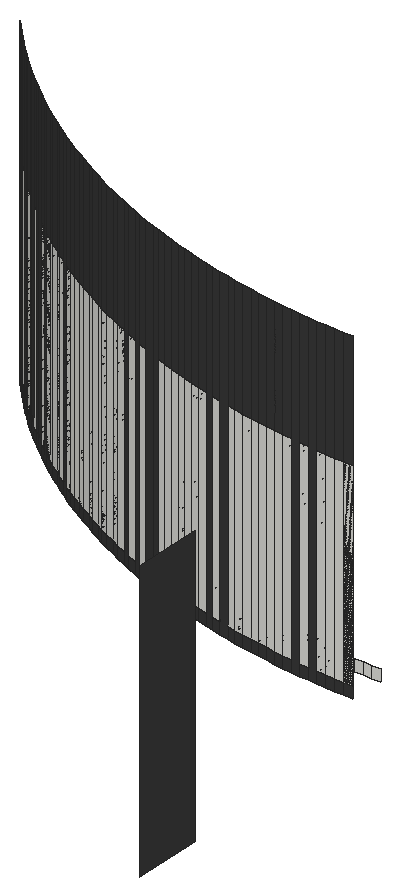
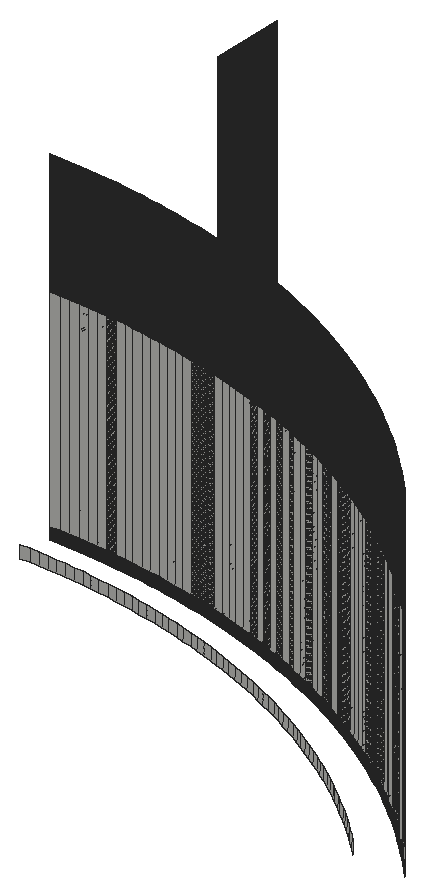
# SketchUp Ruby script. Lengths in inches.
U = 1.inch
M = Sketchup.active_model
def pt(a) = Geom::Point3d.new(a.map { |v| v * U })
def face(e, loops, mat)
  f = e.add_face(loops[0].map { |a| pt(a) })
  loops[1..].each { |l| e.add_face(l.map { |a| pt(a) }).erase! }
  f.material = f.back_material = mat if mat
  f
end
# faces: each face lists its corners as indices into pts; further lists are holes
def faces(e, pts, list, mat = nil) = list.each { |f| face(e, (f[0].is_a?(Array) ? f : [f]).map { |l| l.map { |i| pts[i] } }, mat) }
# xy, xz, yz: faces in a plane at the given z, y or x. An outline is a flat list of corners, or four numbers for a rectangle; further outlines are holes
def ring(l) = l.size == 4 ? [[l[0], l[1]], [l[2], l[1]], [l[2], l[3]], [l[0], l[3]]] : l.each_slice(2).to_a
def flat(e, list, mat, &to3) = list.each { |f| face(e, (f[0].is_a?(Array) ? f : [f]).map { |l| ring(l).map { |u, v| to3.(u, v) } }, mat) }
def xy(e, z, list, mat = nil) = flat(e, list, mat) { |x, y| [x, y, z] }
def xz(e, y, list, mat = nil) = flat(e, list, mat) { |x, z| [x, y, z] }
def yz(e, x, list, mat = nil) = flat(e, list, mat) { |y, z| [x, y, z] }
def lines(e, pts, list) = list.each { |a, b| e.add_line(pt(pts[a]), pt(pts[b])) }
# prism: a flat outline (further loops are holes) pulled along v
def prism(e, loops, v, mat = nil)
  f = face(e, loops, mat); d = Geom::Vector3d.new(v.map { |x| x * U })
  f.pushpull(f.normal.samedirection?(d) ? d.length : -d.length)
end
def box(e, o, s, mat = nil) = prism(e, [[o, [o[0] + s[0], o[1], o[2]], [o[0] + s[0], o[1] + s[1], o[2]], [o[0], o[1] + s[1], o[2]]]], [0, 0, s[2]], mat)
def at(x, y, z, deg = 0) = Geom::Transformation.translation(pt([x, y, z])) * Geom::Transformation.rotation(ORIGIN, Z_AXIS, deg.degrees)
def axes(o, x, y, z) = Geom::Transformation.new([*x, 0, *y, 0, *z, 0, *pt(o).to_a, 1])
def part(name) = M.definitions.add(name)
# library, detail: a bought-in or finely detailed component or shape, given as its bounding box
def library(name, o, s) = part(name).tap { |d| box(d.entities, o, s) }
def detail(e, o, s) = box(e.add_group.entities, o, s)
def put(e, d, t, mat = nil) = e.add_instance(d, t).tap { |i| i.material = mat if mat }
def group(e, t, mat = nil) = e.add_group.tap { |g| g.transformation = t; g.material = mat if mat }.entities
root = M.entities
M.materials.add("1496 AP 8293 CARBON COPY").color = [58, 58, 58]
xz(root,85,[[43.61,129.5,44,138]])
xz(root,85,[[43.61,129,44,143]],"1496 AP 8293 CARBON COPY")
xz(root,86.5,[[43.625,129,44,129.5]])
yz(root,46,[[71,129,74,141]],"1496 AP 8293 CARBON COPY")
p = [[42.43,85.04,129],[42.04,85.0625,129],[42.04,85.0625,143],[42.43,85.04,143],[42.82,85.02,129],[42.82,85.02,143],
  [43.21,85.01,129],[43.21,85.01,143],[43.61,85,129],[43.61,85,143],[41.25,85.125,129],[40.86,85.16,129],
  [40.86,85.16,143],[41.25,85.125,143],[41.65,85.09,129],[41.65,85.09,143],[40.47,85.21,129],[40.08,85.26,129],
  [40.08,85.26,143],[40.47,85.21,143],[39.7,85.31,129],[39.31,85.37,129],[39.31,85.37,143],[39.7,85.31,143],
  [38.92,85.43,129],[38.53,85.5,129],[38.53,85.5,143],[38.92,85.43,143],[38.15,85.58,129],[38.15,85.58,143],
  [37.76,85.66,129],[37.76,85.66,143],[37.38,85.74,129],[37,85.83,129],[37,85.83,143],[37.38,85.74,143],
  [36.62,85.92,129],[36.62,85.92,143],[36.24,86.02,129],[36.24,86.02,143],[35.86,86.125,129],[35.86,86.125,143],
  [35.48,86.24,129],[35.48,86.24,143],[35.1,86.35,129],[35.1,86.35,143],[34.73,86.47,129],[34.73,86.47,143],
  [34.36,86.59,129],[34.36,86.59,143],[42.14,86.5625,129],[42.51,86.54,129],[42.51,86.54,129.5],[42.14,86.5625,129.5],
  [42.88,86.52,129],[42.88,86.52,129.5],[43.25,86.51,129],[43.25,86.51,129.5],[43.625,86.5,129],[43.625,86.5,129.5],
  [33.99,86.72,129],[33.99,86.72,143],[41.02,86.66,129],[41.39,86.62,129],[41.39,86.62,129.5],[41.02,86.66,129.5],
  [41.76,86.59,129],[41.76,86.59,129.5],[33.62,86.85,129],[33.62,86.85,143],[39.91,86.79,129],[40.28,86.74,129],
  [40.28,86.74,129.5],[39.91,86.79,129.5],[40.65,86.7,129],[40.65,86.7,129.5],[39.54,86.85,129],[39.54,86.85,129.5],
  [33.25,86.99,129],[33.25,86.99,143],[38.81,86.98,129],[39.17,86.91,129],[39.17,86.91,129.5],[38.81,86.98,129.5],
  [32.88,87.14,129],[32.88,87.14,143],[38.07,87.12,129],[38.44,87.05,129],[38.44,87.05,129.5],[38.07,87.12,129.5],
  [32.52,87.28,129],[32.52,87.28,143],[37.71,87.2,129],[37.71,87.2,129.5],[37.35,87.29,129],[37.35,87.29,129.5],
  [32.16,87.4375,129],[32.16,87.4375,143],[36.98,87.375,129],[36.98,87.375,129.5],[31.8,87.59,129],[31.8,87.59,143],
  [36.625,87.47,129],[36.625,87.47,129.5],[36.26,87.57,129],[36.26,87.57,129.5],[31.44,87.76,129],[31.44,87.76,143],
  [35.91,87.67,129],[35.91,87.67,129.5],[35.55,87.78,129],[35.55,87.78,129.5],[31.08,87.92,129],[31.08,87.92,143],
  [35.19,87.89,129],[35.19,87.89,129.5],[30.73,88.09,129],[30.73,88.09,143],[34.84,88.01,129],[34.84,88.01,129.5],
  [34.49,88.13,129],[34.49,88.13,129.5],[30.38,88.27,129],[30.38,88.27,143],[34.14,88.26,129],[34.14,88.26,129.5],
  [30.03,88.45,129],[30.03,88.45,143],[33.79,88.39,129],[33.79,88.39,129.5],[33.4375,88.53,129],[33.4375,88.53,129.5],
  [29.69,88.64,129],[29.69,88.64,143],[33.09,88.67,129],[33.09,88.67,129.5],[29.34,88.83,129],[29.34,88.83,143],
  [32.75,88.8125,129],[32.75,88.8125,129.5],[29,89.02,129],[29,89.02,143],[32.41,88.96,129],[32.41,88.96,129.5],
  [28.66,89.22,129],[28.66,89.22,143],[32.07,89.12,129],[32.07,89.12,129.5],[31.73,89.28,129],[31.73,89.28,129.5],
  [28.33,89.42,129],[28.33,89.42,143],[31.39,89.4375,129],[31.39,89.4375,129.5],[27.99,89.63,129],[27.99,89.63,143],
  [31.0625,89.61,129],[31.0625,89.61,129.5],[27.66,89.84,129],[27.66,89.84,143],[30.73,89.78,129],[30.73,89.78,129.5],
  [27.33,90.06,129],[27.33,90.06,143],[30.4,89.95,129],[30.4,89.95,129.5],[30.07,90.13,129],[30.07,90.13,129.5],
  [27.01,90.28,129],[27.01,90.28,143],[29.75,90.32,129],[29.75,90.32,129.5],[26.6875,90.5,129],[26.6875,90.5,143],
  [29.43,90.51,129],[29.43,90.51,129.5],[26.37,90.73,129],[26.37,90.73,143],[29.11,90.7,129],[29.11,90.7,129.5],
  [26.05,90.96,129],[26.05,90.96,143],[28.79,90.9,129],[28.79,90.9,129.5],[28.48,91.1,129],[28.48,91.1,129.5],
  [25.74,91.2,129],[25.74,91.2,143],[28.17,91.3,129],[28.17,91.3,129.5],[25.43,91.44,129],[25.43,91.44,143],
  [27.86,91.51,129],[27.86,91.51,129.5],[25.12,91.6875,129],[25.12,91.6875,143],[27.55,91.73,129],[27.55,91.73,129.5],
  [24.82,91.93,129],[24.82,91.93,143],[27.25,91.94,129],[27.25,91.94,129.5],[24.52,92.1875,129],[24.52,92.1875,143],
  [26.95,92.16,129],[26.95,92.16,129.5],[24.22,92.44,129],[24.22,92.44,143],[26.65,92.39,129],[26.65,92.39,129.5],
  [23.93,92.71,129],[23.93,92.71,143],[26.36,92.62,129],[26.36,92.62,129.5],[26.0625,92.85,129],[26.0625,92.85,129.5],
  [23.64,92.97,129],[23.64,92.97,143],[25.78,93.09,129],[25.78,93.09,129.5],[23.35,93.24,129],[23.35,93.24,143],
  [25.49,93.33,129],[25.49,93.33,129.5],[23.07,93.51,129],[23.07,93.51,143],[25.21,93.57,129],[25.21,93.57,129.5],
  [22.79,93.79,129],[22.79,93.79,143],[24.93,93.82,129],[24.93,93.82,129.5],[22.51,94.07,129],[22.51,94.07,143],
  [24.65,94.07,129],[24.65,94.07,129.5],[22.24,94.35,129],[22.24,94.35,143],[24.38,94.33,129],[24.38,94.33,129.5],
  [21.97,94.64,129],[21.97,94.64,143],[24.11,94.59,129],[24.11,94.59,129.5],[21.71,94.93,129],[21.71,94.93,143],
  [23.85,94.85,129],[23.85,94.85,129.5],[42.43,85.04,138],[42.04,85.0625,138],[42.04,85.0625,129.5],[42.43,85.04,129.5],
  [42.82,85.02,138],[42.82,85.02,129.5],[43.21,85.01,138],[43.21,85.01,129.5],[43.61,85,138],[43.61,85,129.5],
  [41.25,85.125,138],[40.86,85.16,138],[40.86,85.16,129.5],[41.25,85.125,129.5],[41.65,85.09,138],[41.65,85.09,129.5],
  [40.47,85.21,138],[40.08,85.26,138],[40.08,85.26,129.5],[40.47,85.21,129.5],[39.7,85.31,138],[39.31,85.37,138],
  [39.31,85.37,129.5],[39.7,85.31,129.5],[38.92,85.43,138],[38.53,85.5,138],[38.53,85.5,129.5],[38.92,85.43,129.5],
  [38.15,85.58,138],[38.15,85.58,129.5],[37.76,85.66,138],[37.76,85.66,129.5],[37.38,85.74,138],[37,85.83,138],
  [37,85.83,129.5],[37.38,85.74,129.5],[36.62,85.92,138],[36.62,85.92,129.5],[36.24,86.02,138],[36.24,86.02,129.5],
  [35.86,86.125,138],[35.86,86.125,129.5],[35.48,86.24,138],[35.48,86.24,129.5],[35.1,86.35,138],[35.1,86.35,129.5],
  [34.73,86.47,138],[34.73,86.47,129.5],[34.36,86.59,138],[34.36,86.59,129.5],[33.99,86.72,138],[33.99,86.72,129.5],
  [33.62,86.85,138],[33.62,86.85,129.5],[33.25,86.99,138],[33.25,86.99,129.5],[32.88,87.14,138],[32.88,87.14,129.5],
  [32.52,87.28,138],[32.52,87.28,129.5],[32.16,87.4375,138],[32.16,87.4375,129.5],[31.8,87.59,138],[31.8,87.59,129.5],
  [31.44,87.76,138],[31.44,87.76,129.5],[31.08,87.92,138],[31.08,87.92,129.5],[30.73,88.09,138],[30.73,88.09,129.5],
  [30.38,88.27,138],[30.38,88.27,129.5],[30.03,88.45,138],[30.03,88.45,129.5],[29.69,88.64,138],[29.69,88.64,129.5],
  [29.34,88.83,138],[29.34,88.83,129.5],[29,89.02,138],[29,89.02,129.5],[28.66,89.22,138],[28.66,89.22,129.5],
  [28.33,89.42,138],[28.33,89.42,129.5],[27.99,89.63,138],[27.99,89.63,129.5],[27.66,89.84,138],[27.66,89.84,129.5],
  [27.33,90.06,138],[27.33,90.06,129.5],[27.01,90.28,138],[27.01,90.28,129.5],[26.6875,90.5,138],[26.6875,90.5,129.5],
  [26.37,90.73,138],[26.37,90.73,129.5],[26.05,90.96,138],[26.05,90.96,129.5],[25.74,91.2,138],[25.74,91.2,129.5],
  [25.43,91.44,138],[25.43,91.44,129.5],[25.12,91.6875,138],[25.12,91.6875,129.5],[24.82,91.93,138],[24.82,91.93,129.5],
  [24.52,92.1875,138],[24.52,92.1875,129.5],[24.22,92.44,138],[24.22,92.44,129.5],[23.93,92.71,138],[23.93,92.71,129.5],
  [23.64,92.97,138],[23.64,92.97,129.5],[23.35,93.24,138],[23.35,93.24,129.5],[23.07,93.51,138],[23.07,93.51,129.5],
  [22.79,93.79,138],[22.79,93.79,129.5],[22.51,94.07,138],[22.51,94.07,129.5],[22.24,94.35,138],[22.24,94.35,129.5],
  [21.97,94.64,138],[21.97,94.64,129.5],[21.71,94.93,138],[21.71,94.93,129.5]]
faces(root,p,[[0,1,2,3],[4,0,3,5],[6,4,5,7],[8,6,7,9],[10,11,12,13],[14,10,13,15],[1,14,15,2],[16,17,18,19],
  [11,16,19,12],[20,21,22,23],[17,20,23,18],[24,25,26,27],[21,24,27,22],[25,28,29,26],[28,30,31,29],[32,33,34,35],
  [30,32,35,31],[33,36,37,34],[36,38,39,37],[38,40,41,39],[40,42,43,41],[42,44,45,43],[44,46,47,45],[46,48,49,47],
  [48,60,61,49],[60,68,69,61],[68,78,79,69],[78,84,85,79],[84,90,91,85],[90,96,97,91],[96,100,101,97],[100,106,107,101],
  [106,112,113,107],[112,116,117,113],[116,122,123,117],[122,126,127,123],[126,132,133,127],[132,136,137,133],[136,140,141,137],[140,144,145,141],
  [144,150,151,145],[150,154,155,151],[154,158,159,155],[158,162,163,159],[162,168,169,163],[168,172,173,169],[172,176,177,173],[176,180,181,177],
  [180,186,187,181],[186,190,191,187],[190,194,195,191],[194,198,199,195],[198,202,203,199],[202,206,207,203],[206,210,211,207],[210,216,217,211],
  [216,220,221,217],[220,224,225,221],[224,228,229,225],[228,232,233,229],[232,236,237,233],[236,240,241,237],[240,244,245,241]],"1496 AP 8293 CARBON COPY")
faces(root,p,[[50,51,52,53],[51,54,55,52],[54,56,57,55],[56,58,59,57],[62,63,64,65],[63,66,67,64],[66,50,53,67],[70,71,72,73],
  [71,74,75,72],[74,62,65,75],[76,70,73,77],[80,81,82,83],[81,76,77,82],[86,87,88,89],[87,80,83,88],[92,86,89,93],
  [94,92,93,95],[98,94,95,99],[102,98,99,103],[104,102,103,105],[108,104,105,109],[110,108,109,111],[114,110,111,115],[118,114,115,119],
  [120,118,119,121],[124,120,121,125],[128,124,125,129],[130,128,129,131],[134,130,131,135],[138,134,135,139],[142,138,139,143],[146,142,143,147],
  [148,146,147,149],[152,148,149,153],[156,152,153,157],[160,156,157,161],[164,160,161,165],[166,164,165,167],[170,166,167,171],[174,170,171,175],
  [178,174,175,179],[182,178,179,183],[184,182,183,185],[188,184,185,189],[192,188,189,193],[196,192,193,197],[200,196,197,201],[204,200,201,205],
  [208,204,205,209],[212,208,209,213],[214,212,213,215],[218,214,215,219],[222,218,219,223],[226,222,223,227],[230,226,227,231],[234,230,231,235],
  [238,234,235,239],[242,238,239,243],[246,242,243,247],[248,249,250,251],[252,248,251,253],[254,252,253,255],[256,254,255,257],[258,259,260,261],
  [262,258,261,263],[249,262,263,250],[264,265,266,267],[259,264,267,260],[268,269,270,271],[265,268,271,266],[272,273,274,275],[269,272,275,270],
  [273,276,277,274],[276,278,279,277],[280,281,282,283],[278,280,283,279],[281,284,285,282],[284,286,287,285],[286,288,289,287],[288,290,291,289],
  [290,292,293,291],[292,294,295,293],[294,296,297,295],[296,298,299,297],[298,300,301,299],[300,302,303,301],[302,304,305,303],[304,306,307,305],
  [306,308,309,307],[308,310,311,309],[310,312,313,311],[312,314,315,313],[314,316,317,315],[316,318,319,317],[318,320,321,319],[320,322,323,321],
  [322,324,325,323],[324,326,327,325],[326,328,329,327],[328,330,331,329],[330,332,333,331],[332,334,335,333],[334,336,337,335],[336,338,339,337],
  [338,340,341,339],[340,342,343,341],[342,344,345,343],[344,346,347,345],[346,348,349,347],[348,350,351,349],[350,352,353,351],[352,354,355,353],
  [354,356,357,355],[356,358,359,357],[358,360,361,359],[360,362,363,361],[362,364,365,363],[364,366,367,365],[366,368,369,367],[368,370,371,369],
  [370,372,373,371],[372,374,375,373]])
